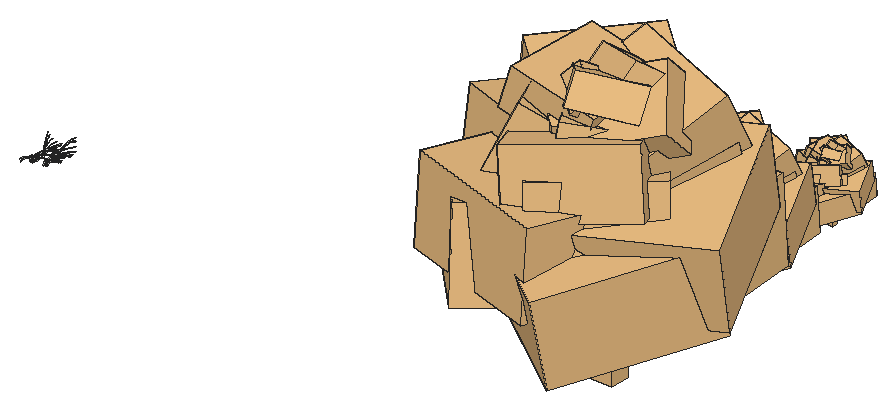
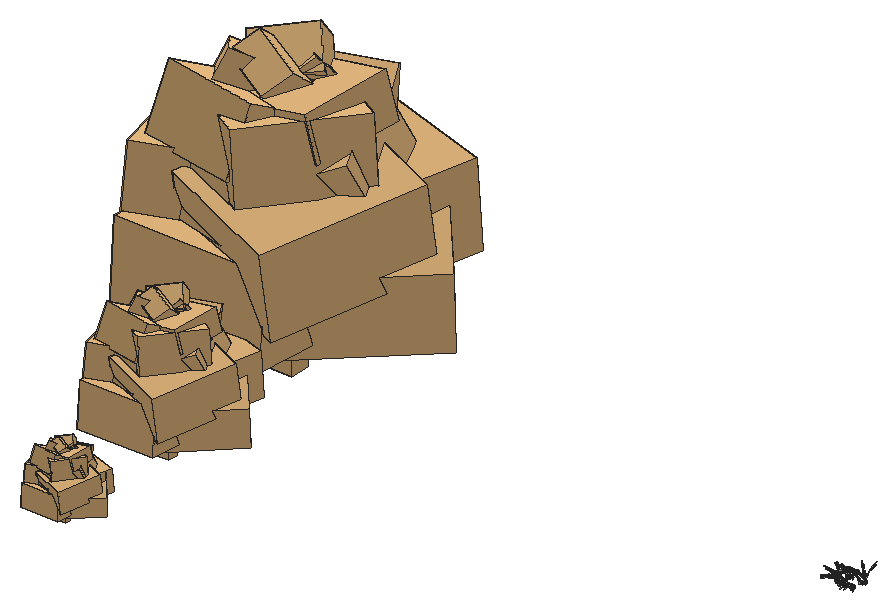
# SketchUp Ruby script. Lengths in inches.
U = 1.inch
M = Sketchup.active_model
def pt(a) = Geom::Point3d.new(a.map { |v| v * U })
def face(e, loops, mat)
  f = e.add_face(loops[0].map { |a| pt(a) })
  loops[1..].each { |l| e.add_face(l.map { |a| pt(a) }).erase! }
  f.material = f.back_material = mat if mat
  f
end
# faces: each face lists its corners as indices into pts; further lists are holes
def faces(e, pts, list, mat = nil) = list.each { |f| face(e, (f[0].is_a?(Array) ? f : [f]).map { |l| l.map { |i| pts[i] } }, mat) }
# xy, xz, yz: faces in a plane at the given z, y or x. An outline is a flat list of corners, or four numbers for a rectangle; further outlines are holes
def ring(l) = l.size == 4 ? [[l[0], l[1]], [l[2], l[1]], [l[2], l[3]], [l[0], l[3]]] : l.each_slice(2).to_a
def flat(e, list, mat, &to3) = list.each { |f| face(e, (f[0].is_a?(Array) ? f : [f]).map { |l| ring(l).map { |u, v| to3.(u, v) } }, mat) }
def xy(e, z, list, mat = nil) = flat(e, list, mat) { |x, y| [x, y, z] }
def xz(e, y, list, mat = nil) = flat(e, list, mat) { |x, z| [x, y, z] }
def yz(e, x, list, mat = nil) = flat(e, list, mat) { |y, z| [x, y, z] }
def lines(e, pts, list) = list.each { |a, b| e.add_line(pt(pts[a]), pt(pts[b])) }
# prism: a flat outline (further loops are holes) pulled along v
def prism(e, loops, v, mat = nil)
  f = face(e, loops, mat); d = Geom::Vector3d.new(v.map { |x| x * U })
  f.pushpull(f.normal.samedirection?(d) ? d.length : -d.length)
end
def box(e, o, s, mat = nil) = prism(e, [[o, [o[0] + s[0], o[1], o[2]], [o[0] + s[0], o[1] + s[1], o[2]], [o[0], o[1] + s[1], o[2]]]], [0, 0, s[2]], mat)
def at(x, y, z, deg = 0) = Geom::Transformation.translation(pt([x, y, z])) * Geom::Transformation.rotation(ORIGIN, Z_AXIS, deg.degrees)
def axes(o, x, y, z) = Geom::Transformation.new([*x, 0, *y, 0, *z, 0, *pt(o).to_a, 1])
def part(name) = M.definitions.add(name)
# library, detail: a bought-in or finely detailed component or shape, given as its bounding box
def library(name, o, s) = part(name).tap { |d| box(d.entities, o, s) }
def detail(e, o, s) = box(e.add_group.entities, o, s)
def put(e, d, t, mat = nil) = e.add_instance(d, t).tap { |i| i.material = mat if mat }
def group(e, t, mat = nil) = e.add_group.tap { |g| g.transformation = t; g.material = mat if mat }.entities
root = M.entities
c1 = library("Pine branch",[-164.19,86.97,62.64],[148.2,83.79,137.08])
c2 = part("Gruppe\#2")
detail(c2.entities,[0.71,-7.7,0],[22.57,19.31,263.85])
c3 = part("Kiefer Pine")
put(c3.entities,c1,axes([141.72,46.52,161.66],[-0.02916,-0.63772,0.00271],[0.15221,-0.00358,0.48358],[-0.6193,0.02915,0.11872]))
put(c3.entities,c1,axes([97.98,30.67,99.84],[-0.47537,-0.59297,0.00413],[0.14389,-0.11021,0.73807],[-0.57526,0.46243,0.1812]))
put(c3.entities,c1,axes([147.43,170.77,85.84],[0.66331,0.36209,0.08066],[-0.16152,0.13314,0.73061],[0.33395,-0.6548,0.19316]))
put(c3.entities,c1,axes([126.12,172.51,50.8],[0.58404,0.48629,0.00413],[-0.11903,0.13668,0.73807],[0.47151,-0.56784,0.1812]))
put(c3.entities,c1,axes([129.28,102.66,199.18],[0.3329,0.20176,-0.07756],[-0.04952,0.23763,0.27741],[0.2165,-0.24552,0.14305]))
put(c3.entities,c1,axes([28.39,91.46,58.6],[-0.71464,0.25212,0.05767],[-0.01186,-0.20123,0.73278],[0.25836,0.68814,0.19316]))
put(c3.entities,c1,axes([152.74,49.28,68.93],[0.33164,-0.67512,0.10878],[0.24998,0.23222,0.67911],[-0.63649,-0.26056,0.32339]))
put(c3.entities,c1,axes([-6.13,166.4,41.09],[-0.38774,0.8952,0.21972],[0.05521,-0.21538,0.97497],[0.92011,0.39016,0.03409]))
put(c3.entities,c1,axes([103.12,114.79,195.58],[-0.35402,0.16187,-0.07756],[-0.18541,-0.24864,0.1992],[0.04135,0.27092,0.22915]))
put(c3.entities,c1,axes([201.4375,150.2,7.87],[0.95266,-0.30403,0],[0.02078,0.06511,0.99766],[-0.30332,-0.95043,0.06835]))
put(c3.entities,c1,axes([149.14,-15.51,56.65],[-0.38076,-0.9108,0.15959],[0.00531,0.17044,0.98535],[-0.92466,0.37603,-0.06006]))
put(c3.entities,c1,axes([123.6,85.97,205.1],[0.23507,-0.19426,-0.06076],[0.16806,0.10538,0.1906],[-0.12474,-0.2241,0.1423]))
put(c3.entities,c1,axes([121.72,132.51,172.5],[0.36293,0.20783,-0.0399],[0.00027,0.10027,0.31921],[0.21403,-0.35254,0.06727]))
put(c3.entities,c1,axes([57.2,144.19,196.7],[-0.28797,0.37098,0.1914],[-0.03125,-0.30847,0.33516],[0.44369,0.21905,0.14782]))
put(c3.entities,c1,axes([93.55,232.34,18.61],[0.58552,0.78879,0.18704],[-0.06218,-0.18635,0.98051],[0.80827,-0.58574,-0.06006]))
put(c3.entities,c1,axes([33.34,105.32,91.71],[-0.72171,0.22385,0.08143],[-0.02606,-0.33247,0.68293],[0.23677,0.64572,0.32339]))
put(c3.entities,c1,axes([227.44,74.67,9.76],[0.6363,-0.72678,0.25867],[-0.14373,0.21775,0.96536],[-0.75793,-0.65144,0.03409]))
put(c3.entities,c1,axes([24.14,28.375,-27.51],[-1,0,0],[0,-0.06835,0.99766],[0,0.99766,0.06835]))
put(c3.entities,c2,at(97.66,98.27,0))
put(root,c3,axes([831.84,982.57,0],[0.375,0,0],[0,0.375,0],[0,0,0.375]))
put(root,c3,axes([795.14,752.84,0],[0.75,0,0],[0,0.75,0],[0,0,0.75]))
put(root,c3,axes([733.29,428.49,0],[1.5,0,0],[0,1.5,0],[0,0,1.5]))
g1 = group(root,at(81.27,576.14,0.02))
p = [[0.76,0.64,0],[0.34,0.29,0],[0,0,1.49],[0.14,0.12,2.99],[0.74,0.63,4.45],[1.8,1.53,5.86],
  [3.28,2.79,7.16],[5.16,4.39,8.33],[7.38,6.28,9.33],[9.89,8.41,10.15],[12.625,10.74,10.77],[15.52,13.2,11.16],
  [18.5,15.73,11.32],[21.5,18.28,11.24],[18.56,15.78,11.26],[15.65,13.31,11.05],[12.84,10.92,10.625],[10.19,8.66,9.99],
  [7.76,6.6,9.16],[5.61,4.77,8.16],[3.79,3.22,7.01],[2.33,1.98,5.73],[1.29,1.09,4.36],[0.67,0.57,2.93],
  [0.49,0.42,1.46]]
faces(g1,p,[[0,1,2,3,4,5,6,7,8,9,10,11,12,13,14,15,16,17,18,19,20,21,22,23,24]])
g2 = group(root,at(85.19,579.84,0.02))
p = [[20.78,-0.12,15.34],[23.91,-0.13,15.75],[20.875,-0.12,15.26],[17.94,-0.1,14.58],[15.15,-0.09,13.72],[12.52,-0.07,12.69],
  [10.09,-0.06,11.5],[7.88,-0.04,10.16],[5.93,-0.03,8.7],[4.24,-0.02,7.11],[2.85,-0.02,5.43],[1.76,-0.01,3.67],
  [0.99,-0.01,1.86],[0.54,0,0],[0,0,0],[0.37,0,1.9],[1.09,-0.01,3.76],[2.16,-0.01,5.57],
  [3.5625,-0.02,7.28],[5.28,-0.03,8.9],[7.3,-0.04,10.39],[9.58,-0.05,11.73],[12.11,-0.07,12.91],[14.84,-0.08,13.91],
  [17.74,-0.1,14.73]]
faces(g2,p,[[0,1,2,3,4,5,6,7,8,9,10,11,12,13,14,15,16,17,18,19,20,21,22,23,24]])
g3 = group(root,at(60.93,560.58,0.02))
p = [[0.99,-0.08,0],[0.44,-0.04,0],[0,0,1.49],[0.18,-0.01,2.99],[0.97,-0.08,4.45],[2.35,-0.19,5.86],
  [4.3,-0.35,7.16],[6.75,-0.55,8.33],[9.66,-0.78,9.33],[12.9375,-1.05,10.15],[16.52,-1.34,10.77],[20.31,-1.64,11.16],
  [24.21,-1.96,11.32],[28.13,-2.27,11.24],[24.28,-1.96,11.26],[20.48,-1.66,11.05],[16.8,-1.36,10.625],[13.33,-1.08,9.99],
  [10.15,-0.82,9.16],[7.34,-0.59,8.16],[4.95,-0.4,7.01],[3.05,-0.25,5.73],[1.68,-0.14,4.36],[0.87,-0.07,2.93],
  [0.64,-0.05,1.46]]
faces(g3,p,[[0,1,2,3,4,5,6,7,8,9,10,11,12,13,14,15,16,17,18,19,20,21,22,23,24]])
g4 = group(root,at(83.26,579.85,0.02))
p = [[20.78,-0.12,12.375],[23.91,-0.13,12.7],[20.875,-0.12,12.31],[17.94,-0.1,11.76],[15.15,-0.09,11.07],[12.52,-0.07,10.23],
  [10.09,-0.06,9.27],[7.88,-0.04,8.2],[5.93,-0.03,7.01],[4.24,-0.02,5.74],[2.85,-0.02,4.38],[1.76,-0.01,2.96],
  [0.99,-0.01,1.5],[0.54,0,0],[0,0,0],[0.37,0,1.53],[1.09,-0.01,3.03],[2.16,-0.01,4.49],
  [3.5625,-0.02,5.875],[5.28,-0.03,7.18],[7.3,-0.04,8.375],[9.58,-0.05,9.46],[12.11,-0.07,10.41],[14.84,-0.08,11.22],
  [17.74,-0.1,11.88]]
faces(g4,p,[[0,1,2,3,4,5,6,7,8,9,10,11,12,13,14,15,16,17,18,19,20,21,22,23,24]])
g5 = group(root,at(79.98,578.16,0.02))
p = [[0.92,-0.01,0],[0.41,0,0],[0,0,1.75],[0.17,0,3.51],[0.91,-0.01,5.24],[2.2,-0.01,6.89],
  [4.02,-0.02,8.42],[6.31,-0.04,9.8],[9.02,-0.05,10.98],[12.09,-0.07,11.95],[15.4375,-0.09,12.67],[18.98,-0.11,13.13],
  [22.625,-0.13,13.32],[26.29,-0.15,13.23],[22.69,-0.13,13.25],[19.14,-0.11,13],[15.7,-0.09,12.5],[12.45,-0.07,11.75],
  [9.49,-0.05,10.78],[6.86,-0.04,9.6],[4.63,-0.03,8.25],[2.85,-0.02,6.75],[1.57,-0.01,5.13],[0.8125,0,3.44],
  [0.6,0,1.72]]
faces(g5,p,[[0,1,2,3,4,5,6,7,8,9,10,11,12,13,14,15,16,17,18,19,20,21,22,23,24]])
g6 = group(root,at(66.33,560.42,0.02))
p = [[14.61,-14.77,15.34],[16.8125,-17,15.75],[14.68,-14.84,15.26],[12.62,-12.76,14.58],[10.65,-10.77,13.72],[8.8,-8.9,12.69],
  [7.09,-7.17,11.5],[5.54,-5.61,10.16],[4.17,-4.22,8.7],[2.98,-3.02,7.11],[2,-2.02,5.43],[1.24,-1.25,3.67],
  [0.69,-0.7,1.86],[0.38,-0.38,0],[0,0,0],[0.26,-0.26,1.9],[0.77,-0.77,3.76],[1.52,-1.54,5.57],
  [2.51,-2.53,7.28],[3.72,-3.76,8.9],[5.13,-5.19,10.39],[6.74,-6.8125,11.73],[8.51,-8.61,12.91],[10.43,-10.55,13.91],
  [12.47,-12.61,14.73]]
faces(g6,p,[[0,1,2,3,4,5,6,7,8,9,10,11,12,13,14,15,16,17,18,19,20,21,22,23,24]])
g7 = group(root,at(82.95,578.81,0.02))
p = [[0.52,0.77,0],[0.23,0.34,0],[0,0,1.75],[0.09,0.14,3.51],[0.51,0.75,5.24],[1.23,1.82,6.89],
  [2.25,3.33,8.42],[3.53,5.23,9.8],[5.05,7.48,10.98],[6.77,10.02,11.95],[8.64,12.8,12.67],[10.62,15.73,13.13],
  [12.66,18.75,13.32],[14.71,21.79,13.23],[12.7,18.81,13.25],[10.71,15.86,13],[8.78,13.01,12.5],[6.97,10.32,11.75],
  [5.31,7.86,10.78],[3.84,5.68,9.6],[2.59,3.84,8.25],[1.6,2.37,6.75],[0.88,1.3,5.13],[0.46,0.67,3.44],
  [0.33,0.49,1.72]]
faces(g7,p,[[0,1,2,3,4,5,6,7,8,9,10,11,12,13,14,15,16,17,18,19,20,21,22,23,24]])
g8 = group(root,at(64.97,561.8,0.02))
p = [[14.61,-14.77,12.375],[16.8125,-17,12.7],[14.68,-14.84,12.31],[12.62,-12.76,11.76],[10.65,-10.77,11.07],[8.8,-8.9,10.23],
  [7.09,-7.17,9.27],[5.54,-5.61,8.2],[4.17,-4.22,7.01],[2.98,-3.02,5.74],[2,-2.02,4.38],[1.24,-1.25,2.96],
  [0.69,-0.7,1.5],[0.38,-0.38,0],[0,0,0],[0.26,-0.26,1.53],[0.77,-0.77,3.03],[1.52,-1.54,4.49],
  [2.51,-2.53,5.875],[3.72,-3.76,7.18],[5.13,-5.19,8.375],[6.74,-6.8125,9.46],[8.51,-8.61,10.41],[10.43,-10.55,11.22],
  [12.47,-12.61,11.88]]
faces(g8,p,[[0,1,2,3,4,5,6,7,8,9,10,11,12,13,14,15,16,17,18,19,20,21,22,23,24]])
g9 = group(root,at(61.45,562.93,0.02))
p = [[0.65,-0.66,0],[0.29,-0.29,0],[0,0,1.75],[0.12,-0.12,3.51],[0.64,-0.64,5.24],[1.55,-1.5625,6.89],
  [2.82,-2.86,8.42],[4.4375,-4.49,9.8],[6.35,-6.42,10.98],[8.5,-8.6,11.95],[10.85,-10.98,12.67],[13.34,-13.49,13.13],
  [15.91,-16.09,13.32],[18.48,-18.69,13.23],[15.96,-16.14,13.25],[13.45,-13.61,13],[11.04,-11.16,12.5],[8.76,-8.86,11.75],
  [6.67,-6.74,10.78],[4.82,-4.875,9.6],[3.25,-3.29,8.25],[2.01,-2.03,6.75],[1.11,-1.12,5.13],[0.57,-0.58,3.44],
  [0.42,-0.42,1.72]]
faces(g9,p,[[0,1,2,3,4,5,6,7,8,9,10,11,12,13,14,15,16,17,18,19,20,21,22,23,24]])
g10 = group(root,at(84.27,579.48,0.02))
p = [[0.35,0.86,0],[0.16,0.38,0],[0,0,2.37],[0.0625,0.15,4.75],[0.35,0.84,7.08],[0.84,2.03,9.32],
  [1.53,3.71,11.39],[2.4,5.83,13.25],[3.4375,8.34,14.85],[4.61,11.18,16.15],[5.88,14.27,17.13],[7.23,17.55,17.75],
  [8.62,20.92,18.01],[10.02,24.3,17.89],[8.65,20.98,17.91],[7.29,17.69,17.58],[5.98,14.51,16.9],[4.75,11.52,15.89],
  [3.61,8.77,14.58],[2.61,6.34,12.99],[1.76,4.28,11.15],[1.09,2.64,9.125],[0.6,1.45,6.94],[0.31,0.75,4.66],
  [0.23,0.55,2.33]]
faces(g10,p,[[0,1,2,3,4,5,6,7,8,9,10,11,12,13,14,15,16,17,18,19,20,21,22,23,24]])
g11 = group(root,at(64.02,561.29,0.02))
p = [[0.91,0.18,0],[0.4,0.08,0],[0,0,1.75],[0.16,0.03,3.51],[0.89,0.17,5.24],[2.16,0.42,6.89],
  [3.94,0.76,8.42],[6.19,1.2,9.8],[8.86,1.72,10.98],[11.87,2.3,11.95],[15.16,2.94,12.67],[18.63,3.61,13.13],
  [22.21,4.31,13.32],[25.81,5.01,13.23],[22.28,4.32,13.25],[18.79,3.64,13],[15.41,2.99,12.5],[12.23,2.37,11.75],
  [9.3125,1.81,10.78],[6.73,1.31,9.6],[4.54,0.88,8.25],[2.8,0.54,6.75],[1.54,0.3,5.13],[0.8,0.16,3.44],
  [0.59,0.11,1.72]]
faces(g11,p,[[0,1,2,3,4,5,6,7,8,9,10,11,12,13,14,15,16,17,18,19,20,21,22,23,24]])
g12 = group(root,at(65.42,560.83,0.02))
p = [[0.85,0.36,0],[0.38,0.16,0],[0,0,2.37],[0.15,0.0625,4.75],[0.84,0.35,7.08],[2.03,0.85,9.32],
  [3.71,1.54,11.39],[5.83,2.42,13.25],[8.33,3.47,14.85],[11.16,4.65,16.15],[14.25,5.93,17.13],[17.52,7.29,17.75],
  [20.89,8.69,18.01],[24.27,10.1,17.89],[20.95,8.72,17.91],[17.67,7.35,17.58],[14.49,6.03,16.9],[11.5,4.79,15.89],
  [8.76,3.65,14.58],[6.33,2.63,12.99],[4.27,1.78,11.15],[2.63,1.1,9.125],[1.45,0.6,6.94],[0.75,0.3125,4.66],
  [0.55,0.23,2.33]]
faces(g12,p,[[0,1,2,3,4,5,6,7,8,9,10,11,12,13,14,15,16,17,18,19,20,21,22,23,24]])
g13 = group(root,at(83.21,584.52,0.02))
p = [[7.92,19.21,20.75],[9.11,22.11,21.3],[7.96,19.3,20.63],[6.84,16.59,19.72],[5.77,14.01,18.55],[4.77,11.58,17.16],
  [3.85,9.33,15.55],[3,7.29,13.74],[2.26,5.48,11.76],[1.62,3.92,9.62],[1.09,2.63,7.35],[0.67,1.625,4.97],
  [0.375,0.91,2.51],[0.21,0.5,0],[0,0,0],[0.14,0.34,2.57],[0.41,1.01,5.09],[0.82,2,7.53],
  [1.36,3.3,9.85],[2.01,4.89,12.03],[2.78,6.75,14.04],[3.65,8.86,15.86],[4.61,11.19,17.46],[5.65,13.72,18.82],
  [6.76,16.4,19.92]]
faces(g13,p,[[0,1,2,3,4,5,6,7,8,9,10,11,12,13,14,15,16,17,18,19,20,21,22,23,24]])
g14 = group(root,at(84.5625,577.8,0.02))
p = [[16.41,-12.74,15.34],[18.89,-14.66,15.75],[16.49,-12.8,15.26],[14.17,-11,14.58],[11.97,-9.29,13.72],[9.89,-7.68,12.69],
  [7.97,-6.1875,11.5],[6.23,-4.83,10.16],[4.68,-3.64,8.7],[3.35,-2.6,7.11],[2.25,-1.75,5.43],[1.39,-1.08,3.67],
  [0.78,-0.6,1.86],[0.43,-0.33,0],[0,0,0],[0.29,-0.22,1.9],[0.86,-0.67,3.76],[1.71,-1.32,5.57],
  [2.82,-2.1875,7.28],[4.17,-3.24,8.9],[5.77,-4.48,10.39],[7.57,-5.875,11.73],[9.5625,-7.42,12.91],[11.72,-9.1,13.91],
  [14.01,-10.88,14.73]]
faces(g14,p,[[0,1,2,3,4,5,6,7,8,9,10,11,12,13,14,15,16,17,18,19,20,21,22,23,24]])
g15 = group(root,at(78.09,577.63,0.02))
p = [[0.71,0.27,0],[0.31,0.12,0],[0,0,1.24],[0.13,0.05,2.49],[0.69,0.27,3.72],[1.68,0.65,4.89],
  [3.07,1.18,5.98],[4.83,1.85,6.95],[6.91,2.65,7.8],[9.26,3.55,8.48],[11.82,4.53,8.99],[14.53,5.57,9.32],
  [17.32,6.64,9.46],[20.125,7.72,9.39],[17.375,6.66,9.4],[14.65,5.62,9.23],[12.02,4.61,8.875],[9.54,3.66,8.35],
  [7.26,2.78,7.65],[5.25,2.01,6.82],[3.54,1.36,5.86],[2.18,0.84,4.79],[1.2,0.46,3.64],[0.625,0.24,2.45],
  [0.46,0.18,1.22]]
faces(g15,p,[[0,1,2,3,4,5,6,7,8,9,10,11,12,13,14,15,16,17,18,19,20,21,22,23,24]])
g16 = group(root,at(82.47,582.74,0.02))
p = [[7.92,19.21,16.73],[9.11,22.11,17.17],[7.96,19.3,16.64],[6.84,16.59,15.9],[5.77,14.01,14.96],[4.77,11.58,13.84],
  [3.85,9.33,12.54],[3,7.29,11.08],[2.26,5.48,9.48],[1.62,3.92,7.76],[1.09,2.63,5.92],[0.67,1.625,4.01],
  [0.375,0.91,2.02],[0.21,0.5,0],[0,0,0],[0.14,0.34,2.07],[0.41,1.01,4.1],[0.82,2,6.07],
  [1.36,3.3,7.94],[2.01,4.89,9.7],[2.78,6.75,11.33],[3.65,8.86,12.79],[4.61,11.19,14.08],[5.65,13.72,15.17],
  [6.76,16.4,16.0625]]
faces(g16,p,[[0,1,2,3,4,5,6,7,8,9,10,11,12,13,14,15,16,17,18,19,20,21,22,23,24]])
g17 = group(root,at(66.16,578.48,0.02))
p = [[0.07,0.81,0],[0.03,0.36,0],[0,0,1.23],[0.01,0.15,2.46],[0.0625,0.8,3.67],[0.16,1.9375,4.82],
  [0.29,3.54,5.89],[0.45,5.56,6.85],[0.64,7.95,7.68],[0.86,10.65,8.36],[1.1,13.6,8.86],[1.35,16.71,9.18],
  [1.61,19.92,9.32],[1.87,23.15,9.25],[1.62,19.98,9.27],[1.36,16.85,9.09],[1.12,13.82,8.74],[0.89,10.97,8.22],
  [0.68,8.35,7.54],[0.49,6.04,6.72],[0.33,4.08,5.77],[0.2,2.51,4.72],[0.11,1.38,3.59],[0.06,0.72,2.41],
  [0.04,0.53,1.2]]
faces(g17,p,[[0,1,2,3,4,5,6,7,8,9,10,11,12,13,14,15,16,17,18,19,20,21,22,23,24]])
g18 = group(root,at(68.24,565.14,0.02))
p = [[19.18,7.98,20.75],[22.08,9.1875,21.3],[19.27,8.02,20.63],[16.57,6.9,19.72],[13.98,5.82,18.55],[11.56,4.8125,17.16],
  [9.32,3.88,15.55],[7.28,3.03,13.74],[5.47,2.28,11.76],[3.92,1.63,9.62],[2.63,1.09,7.35],[1.625,0.68,4.97],
  [0.91,0.38,2.51],[0.5,0.21,0],[0,0,0],[0.34,0.14,2.57],[1.01,0.42,5.09],[1.99,0.83,7.53],
  [3.29,1.37,9.85],[4.88,2.03,12.03],[6.74,2.81,14.04],[8.85,3.68,15.86],[11.18,4.65,17.46],[13.7,5.7,18.82],
  [16.375,6.82,19.92]]
faces(g18,p,[[0,1,2,3,4,5,6,7,8,9,10,11,12,13,14,15,16,17,18,19,20,21,22,23,24]])
g19 = group(root,at(83.04,578.98,0.02))
p = [[16.41,-12.74,12.375],[18.89,-14.66,12.7],[16.49,-12.8,12.31],[14.17,-11,11.76],[11.97,-9.29,11.07],[9.89,-7.68,10.23],
  [7.97,-6.1875,9.27],[6.23,-4.83,8.2],[4.68,-3.64,7.01],[3.35,-2.6,5.74],[2.25,-1.75,4.38],[1.39,-1.08,2.96],
  [0.78,-0.6,1.5],[0.43,-0.33,0],[0,0,0],[0.29,-0.22,1.53],[0.86,-0.67,3.03],[1.71,-1.32,4.49],
  [2.82,-2.1875,5.875],[4.17,-3.24,7.18],[5.77,-4.48,8.375],[7.57,-5.875,9.46],[9.5625,-7.42,10.41],[11.72,-9.1,11.22],
  [14.01,-10.88,11.88]]
faces(g19,p,[[0,1,2,3,4,5,6,7,8,9,10,11,12,13,14,15,16,17,18,19,20,21,22,23,24]])
g20 = group(root,at(64.4375,559.43,0.02))
p = [[2.6,-20.61,15.34],[2.99,-23.72,15.75],[2.61,-20.71,15.26],[2.24,-17.8,14.58],[1.89,-15.03,13.72],[1.56,-12.42,12.69],
  [1.26,-10.01,11.5],[0.99,-7.82,10.16],[0.74,-5.88,8.7],[0.53,-4.21,7.11],[0.36,-2.83,5.43],[0.22,-1.74,3.67],
  [0.125,-0.98,1.86],[0.07,-0.54,0],[0,0,0],[0.05,-0.36,1.9],[0.14,-1.08,3.76],[0.27,-2.14,5.57],
  [0.45,-3.54,7.28],[0.66,-5.24,8.9],[0.91,-7.24,10.39],[1.2,-9.51,11.73],[1.51,-12.01,12.91],[1.85,-14.72,13.91],
  [2.22,-17.6,14.73]]
faces(g20,p,[[0,1,2,3,4,5,6,7,8,9,10,11,12,13,14,15,16,17,18,19,20,21,22,23,24]])
g21 = group(root,at(79.64,581.62,0.02))
p = [[0.78,-0.61,0],[0.35,-0.27,0],[0,0,1.49],[0.14,-0.11,2.99],[0.77,-0.6,4.45],[1.87,-1.45,5.86],
  [3.41,-2.64,7.16],[5.35,-4.15,8.33],[7.65,-5.94,9.33],[10.25,-7.96,10.15],[13.09,-10.16,10.77],[16.09,-12.49,11.16],
  [19.18,-14.89,11.32],[22.29,-17.3,11.24],[19.24,-14.9375,11.26],[16.23,-12.6,11.05],[13.3125,-10.33,10.625],[10.5625,-8.2,9.99],
  [8.04,-6.24,9.16],[5.8125,-4.51,8.16],[3.93,-3.05,7.01],[2.42,-1.88,5.73],[1.33,-1.04,4.36],[0.69,-0.54,2.93],
  [0.51,-0.39,1.46]]
faces(g21,p,[[0,1,2,3,4,5,6,7,8,9,10,11,12,13,14,15,16,17,18,19,20,21,22,23,24]])
g22 = group(root,at(66.3,582.92,0.02))
p = [[12.16,12.02,12.63],[13.99,13.84,12.96],[12.22,12.08,12.56],[10.5,10.38,12],[8.86,8.77,11.29],[7.33,7.25,10.44],
  [5.9,5.84,9.46],[4.61,4.5625,8.36],[3.47,3.43,7.16],[2.48,2.46,5.85],[1.67,1.65,4.47],[1.03,1.02,3.02],
  [0.58,0.57,1.53],[0.32,0.3125,0],[0,0,0],[0.21,0.21,1.5625],[0.64,0.63,3.1],[1.26,1.25,4.58],
  [2.09,2.0625,6],[3.09,3.06,7.32],[4.27,4.22,8.55],[5.61,5.55,9.65],[7.08,7.01,10.625],[8.68,8.59,11.45],
  [10.38,10.27,12.12]]
faces(g22,p,[[0,1,2,3,4,5,6,7,8,9,10,11,12,13,14,15,16,17,18,19,20,21,22,23,24]])
g23 = group(root,at(81.09,560.69,0.02))
p = [[0.67,0.57,0],[0.3,0.25,0],[0,0,1.32],[0.12,0.1,2.64],[0.66,0.56,3.94],[1.59,1.35,5.18],
  [2.91,2.47,6.33],[4.57,3.88,7.37],[6.53,5.55,8.26],[8.75,7.44,8.99],[11.17,9.5,9.53],[13.73,11.68,9.875],
  [16.37,13.92,10.02],[19.02,16.18,9.95],[16.42,13.97,9.96],[13.85,11.78,9.78],[11.36,9.66,9.4],[9.01,7.67,8.84],
  [6.86,5.84,8.11],[4.96,4.22,7.22],[3.35,2.85,6.2],[2.07,1.76,5.07],[1.14,0.97,3.86],[0.59,0.5,2.59],
  [0.43,0.37,1.29]]
faces(g23,p,[[0,1,2,3,4,5,6,7,8,9,10,11,12,13,14,15,16,17,18,19,20,21,22,23,24]])
g24 = group(root,at(59.74,563.88,0.02))
p = [[0.69,-0.31,0],[0.31,-0.14,0],[0,0,1.24],[0.125,-0.06,2.49],[0.68,-0.3,3.72],[1.65,-0.73,4.89],
  [3.01,-1.34,5.98],[4.73,-2.11,6.95],[6.76,-3.01,7.8],[9.06,-4.04,8.48],[11.5625,-5.15,8.99],[14.21,-6.33,9.32],
  [16.94,-7.55,9.46],[19.6875,-8.77,9.39],[17,-7.58,9.4],[14.33,-6.39,9.23],[11.76,-5.24,8.875],[9.33,-4.16,8.35],
  [7.1,-3.17,7.65],[5.14,-2.29,6.82],[3.47,-1.55,5.86],[2.14,-0.95,4.79],[1.18,-0.52,3.64],[0.61,-0.27,2.45],
  [0.45,-0.2,1.22]]
faces(g24,p,[[0,1,2,3,4,5,6,7,8,9,10,11,12,13,14,15,16,17,18,19,20,21,22,23,24]])
g25 = group(root,at(66.45,564.4,0.02))
p = [[19.18,7.98,16.73],[22.08,9.1875,17.17],[19.27,8.02,16.64],[16.57,6.9,15.9],[13.98,5.82,14.96],[11.56,4.8125,13.84],
  [9.32,3.88,12.54],[7.28,3.03,11.08],[5.47,2.28,9.48],[3.92,1.63,7.76],[2.63,1.09,5.92],[1.625,0.68,4.01],
  [0.91,0.38,2.02],[0.5,0.21,0],[0,0,0],[0.34,0.14,2.07],[1.01,0.42,4.1],[1.99,0.83,6.07],
  [3.29,1.37,7.94],[4.88,2.03,9.7],[6.74,2.81,11.33],[8.85,3.68,12.79],[11.18,4.65,14.08],[13.7,5.7,15.17],
  [16.375,6.82,16.0625]]
faces(g25,p,[[0,1,2,3,4,5,6,7,8,9,10,11,12,13,14,15,16,17,18,19,20,21,22,23,24]])
g26 = group(root,at(84.5625,563.97,0.02))
p = [[18.39,-0.1,13.58],[21.16,-0.12,13.9375],[18.47,-0.1,13.5],[15.88,-0.09,12.9],[13.41,-0.08,12.14],[11.08,-0.0625,11.23],
  [8.93,-0.05,10.18],[6.98,-0.04,8.99],[5.25,-0.03,7.7],[3.75,-0.02,6.29],[2.52,-0.01,4.81],[1.56,-0.01,3.25],
  [0.87,0,1.64],[0.48,0,0],[0,0,0],[0.32,0,1.68],[0.96,-0.01,3.33],[1.91,-0.01,4.92],
  [3.15,-0.02,6.45],[4.68,-0.03,7.875],[6.46,-0.04,9.19],[8.48,-0.05,10.38],[10.71,-0.06,11.43],[13.13,-0.07,12.3125],
  [15.7,-0.09,13.03]]
faces(g26,p,[[0,1,2,3,4,5,6,7,8,9,10,11,12,13,14,15,16,17,18,19,20,21,22,23,24]])
g27 = group(root,at(65.17,581.8,0.02))
p = [[12.16,12.02,10.18],[13.99,13.84,10.45],[12.22,12.08,10.13],[10.5,10.38,9.68],[8.86,8.77,9.11],[7.33,7.25,8.42],
  [5.9,5.84,7.63],[4.61,4.5625,6.75],[3.47,3.43,5.77],[2.48,2.46,4.72],[1.67,1.65,3.61],[1.03,1.02,2.4375],
  [0.58,0.57,1.23],[0.32,0.3125,0],[0,0,0],[0.21,0.21,1.26],[0.64,0.63,2.5],[1.26,1.25,3.69],
  [2.09,2.0625,4.83],[3.09,3.06,5.91],[4.27,4.22,6.89],[5.61,5.55,7.78],[7.08,7.01,8.57],[8.68,8.59,9.24],
  [10.38,10.27,9.78]]
faces(g27,p,[[0,1,2,3,4,5,6,7,8,9,10,11,12,13,14,15,16,17,18,19,20,21,22,23,24]])
g28 = group(root,at(64.2,561.34,0.02))
p = [[2.6,-20.61,12.375],[2.99,-23.72,12.7],[2.61,-20.71,12.31],[2.24,-17.8,11.76],[1.89,-15.03,11.07],[1.56,-12.42,10.23],
  [1.26,-10.01,9.27],[0.99,-7.82,8.2],[0.74,-5.88,7.01],[0.53,-4.21,5.74],[0.36,-2.83,4.38],[0.22,-1.74,2.96],
  [0.125,-0.98,1.5],[0.07,-0.54,0],[0,0,0],[0.05,-0.36,1.53],[0.14,-1.08,3.03],[0.27,-2.14,4.49],
  [0.45,-3.54,5.875],[0.66,-5.24,7.18],[0.91,-7.24,8.375],[1.2,-9.51,9.46],[1.51,-12.01,10.41],[1.85,-14.72,11.22],
  [2.22,-17.6,11.88]]
faces(g28,p,[[0,1,2,3,4,5,6,7,8,9,10,11,12,13,14,15,16,17,18,19,20,21,22,23,24]])
g29 = group(root,at(64.24,578.9,0.02))
p = [[0.54,0.54,0],[0.24,0.24,0],[0,0,1.44],[0.1,0.1,2.89],[0.53,0.52,4.3125],[1.29,1.27,5.67],
  [2.35,2.32,6.93],[3.69,3.65,8.0625],[5.28,5.22,9.04],[7.08,7,9.83],[9.03,8.93,10.43],[11.11,10.98,10.81],
  [13.24,13.09,10.96],[15.38,15.21,10.89],[13.28,13.13,10.9],[11.2,11.07,10.7],[9.1875,9.08,10.29],[7.29,7.21,9.67],
  [5.55,5.49,8.875],[4.01,3.97,7.9],[2.71,2.68,6.79],[1.67,1.65,5.55],[0.92,0.91,4.22],[0.48,0.47,2.83],
  [0.35,0.35,1.42]]
faces(g29,p,[[0,1,2,3,4,5,6,7,8,9,10,11,12,13,14,15,16,17,18,19,20,21,22,23,24]])
g30 = group(root,at(63.66,565.62,0.02))
p = [[0.125,-0.99,0],[0.06,-0.4375,0],[0,0,1.49],[0.02,-0.18,2.99],[0.12,-0.96,4.45],[0.3,-2.34,5.86],
  [0.54,-4.28,7.16],[0.85,-6.72,8.33],[1.21,-9.61,9.33],[1.62,-12.88,10.15],[2.07,-16.44,10.77],[2.55,-20.21,11.16],
  [3.03,-24.1,11.32],[3.53,-28,11.24],[3.04,-24.17,11.26],[2.57,-20.38,11.05],[2.11,-16.72,10.625],[1.67,-13.27,9.99],
  [1.27,-10.1,9.16],[0.92,-7.3,8.16],[0.62,-4.93,7.01],[0.38,-3.04,5.73],[0.21,-1.67,4.36],[0.11,-0.87,2.93],
  [0.08,-0.64,1.46]]
faces(g30,p,[[0,1,2,3,4,5,6,7,8,9,10,11,12,13,14,15,16,17,18,19,20,21,22,23,24]])
g31 = group(root,at(82.85,563.98,0.02))
p = [[18.39,-0.1,10.95],[21.16,-0.12,11.24],[18.47,-0.1,10.89],[15.88,-0.09,10.41],[13.41,-0.08,9.79],[11.08,-0.0625,9.06],
  [8.93,-0.05,8.21],[6.98,-0.04,7.25],[5.25,-0.03,6.21],[3.75,-0.02,5.08],[2.52,-0.01,3.875],[1.56,-0.01,2.62],
  [0.87,0,1.32],[0.48,0,0],[0,0,0],[0.32,0,1.36],[0.96,-0.01,2.69],[1.91,-0.01,3.97],
  [3.15,-0.02,5.2],[4.68,-0.03,6.35],[6.46,-0.04,7.41],[8.48,-0.05,8.37],[10.71,-0.06,9.21],[13.13,-0.07,9.93],
  [15.7,-0.09,10.51]]
faces(g31,p,[[0,1,2,3,4,5,6,7,8,9,10,11,12,13,14,15,16,17,18,19,20,21,22,23,24]])
g32 = group(root,at(65.59,581.02,0.02))
p = [[-0.14,0.75,0],[-0.0625,0.33,0],[0,0,1.44],[-0.03,0.13,2.89],[-0.14,0.73,4.3125],[-0.34,1.78,5.67],
  [-0.63,3.24,6.93],[-0.99,5.1,8.0625],[-1.41,7.29,9.04],[-1.9,9.77,9.83],[-2.42,12.47,10.43],[-2.97,15.33,10.81],
  [-3.55,18.28,10.96],[-4.12,21.24,10.89],[-3.56,18.33,10.9],[-3,15.46,10.7],[-2.46,12.68,10.29],[-1.95,10.0625,9.67],
  [-1.49,7.66,8.875],[-1.07,5.54,7.9],[-0.73,3.74,6.79],[-0.45,2.31,5.55],[-0.25,1.27,4.22],[-0.13,0.66,2.83],
  [-0.09,0.48,1.42]]
faces(g32,p,[[0,1,2,3,4,5,6,7,8,9,10,11,12,13,14,15,16,17,18,19,20,21,22,23,24]])
g33 = group(root,at(79.94,562.48,0.02))
p = [[0.82,0,0],[0.36,0,0],[0,0,1.55],[0.15,0,3.11],[0.8,0,4.64],[1.95,-0.01,6.1],
  [3.55,-0.02,7.45],[5.58,-0.03,8.67],[7.99,-0.04,9.72],[10.7,-0.06,10.57],[13.66,-0.08,11.21],[16.79,-0.09,11.62],
  [20.02,-0.11,11.79],[23.26,-0.13,11.71],[20.08,-0.11,11.72],[16.93,-0.1,11.5],[13.89,-0.08,11.0625],[11.02,-0.0625,10.4],
  [8.39,-0.05,9.54],[6.07,-0.03,8.5],[4.1,-0.02,7.3],[2.53,-0.01,5.97],[1.39,-0.01,4.54],[0.72,0,3.05],
  [0.53,0,1.52]]
faces(g33,p,[[0,1,2,3,4,5,6,7,8,9,10,11,12,13,14,15,16,17,18,19,20,21,22,23,24]])
g34 = group(root,at(65.96,582.17,0.02))
p = [[-0.29,0.7,0],[-0.13,0.3125,0],[0,0,1.95],[-0.05,0.125,3.91],[-0.29,0.6875,5.83],[-0.7,1.67,7.67],
  [-1.27,3.05,9.37],[-2,4.79,10.9],[-2.85,6.86,12.22],[-3.82,9.1875,13.3],[-4.88,11.73,14.1],[-6,14.42,14.61],
  [-7.16,17.19,14.82],[-8.3125,19.97,14.72],[-7.18,17.24,14.74],[-6.05,14.54,14.47],[-4.96,11.93,13.91],[-3.9375,9.46,13.08],
  [-3,7.21,12],[-2.17,5.21,10.6875],[-1.46,3.52,9.18],[-0.9,2.17,7.51],[-0.5,1.19,5.71],[-0.26,0.62,3.83],
  [-0.1875,0.45,1.91]]
faces(g34,p,[[0,1,2,3,4,5,6,7,8,9,10,11,12,13,14,15,16,17,18,19,20,21,22,23,24]])
g35 = group(root,at(82.57,563.0625,0.02))
p = [[0.46,0.68,0],[0.2,0.3,0],[0,0,1.55],[0.08,0.12,3.11],[0.45,0.66,4.64],[1.09,1.61,6.1],
  [1.99,2.95,7.45],[3.125,4.63,8.67],[4.47,6.62,9.72],[5.99,8.87,10.57],[7.64,11.32,11.21],[9.4,13.92,11.62],
  [11.2,16.59,11.79],[13.02,19.28,11.71],[11.24,16.64,11.72],[9.47,14.04,11.5],[7.77,11.51,11.0625],[6.17,9.14,10.4],
  [4.7,6.96,9.54],[3.39,5.03,8.5],[2.29,3.4,7.3],[1.41,2.09,5.97],[0.78,1.15,4.54],[0.4,0.6,3.05],
  [0.3,0.4375,1.52]]
faces(g35,p,[[0,1,2,3,4,5,6,7,8,9,10,11,12,13,14,15,16,17,18,19,20,21,22,23,24]])
g36 = group(root,at(83.74,563.65,0.02))
p = [[0.3125,0.76,0],[0.14,0.34,0],[0,0,2.1],[0.06,0.14,4.2],[0.31,0.74,6.27],[0.74,1.8,8.24],
  [1.35,3.29,10.08],[2.13,5.16,11.72],[3.04,7.38,13.14],[4.08,9.89,14.3],[5.21,12.63,15.16],[6.4,15.53,15.71],
  [7.63,18.51,15.9375],[8.86,21.51,15.83],[7.65,18.57,15.85],[6.45,15.66,15.56],[5.29,12.84,14.96],[4.2,10.19,14.07],
  [3.2,7.76,12.9],[2.3125,5.61,11.49],[1.5625,3.79,9.87],[0.96,2.33,8.07],[0.53,1.29,6.14],[0.27,0.67,4.12],
  [0.2,0.49,2.06]]
faces(g36,p,[[0,1,2,3,4,5,6,7,8,9,10,11,12,13,14,15,16,17,18,19,20,21,22,23,24]])
g37 = group(root,at(78.07,576.12,0.02))
p = [[0.73,-0.57,0],[0.32,-0.25,0],[0,0,1.75],[0.13,-0.1,3.51],[0.72,-0.56,5.24],[1.74,-1.35,6.89],
  [3.17,-2.46,8.42],[4.98,-3.87,9.8],[7.13,-5.53,10.98],[9.55,-7.42,11.95],[12.19,-9.47,12.67],[14.99,-11.64,13.13],
  [17.87,-13.875,13.32],[20.76,-16.12,13.23],[17.93,-13.92,13.25],[15.12,-11.73,13],[12.4,-9.625,12.5],[9.84,-7.64,11.75],
  [7.49,-5.82,10.78],[5.42,-4.2,9.6],[3.66,-2.84,8.25],[2.25,-1.75,6.75],[1.24,-0.96,5.13],[0.64,-0.5,3.44],
  [0.47,-0.37,1.72]]
faces(g37,p,[[0,1,2,3,4,5,6,7,8,9,10,11,12,13,14,15,16,17,18,19,20,21,22,23,24]])
g38 = group(root,at(74.27,585.01,0.02))
p = [[18.35,-9.75,14.56],[21.11,-11.23,14.94],[18.43,-9.8,14.48],[15.84,-8.42,13.83],[13.375,-7.11,13.02],[11.05,-5.88,12.04],
  [8.91,-4.74,10.91],[6.96,-3.7,9.64],[5.23,-2.78,8.25],[3.75,-1.99,6.75],[2.51,-1.34,5.15],[1.55,-0.83,3.49],
  [0.87,-0.46,1.76],[0.48,-0.25,0],[0,0,0],[0.32,-0.17,1.8],[0.96,-0.51,3.57],[1.91,-1.01,5.28],
  [3.15,-1.67,6.91],[4.67,-2.48,8.44],[6.45,-3.43,9.85],[8.46,-4.5,11.13],[10.6875,-5.68,12.25],[13.1,-6.97,13.2],
  [15.66,-8.33,13.97]]
faces(g38,p,[[0,1,2,3,4,5,6,7,8,9,10,11,12,13,14,15,16,17,18,19,20,21,22,23,24]])
g39 = group(root,at(62.41,584.49,0.02))
p = [[-6.57,15.79,17.08],[-7.5625,18.17,17.53],[-6.6,15.86,16.98],[-5.68,13.63,16.23],[-4.79,11.51,15.27],[-3.96,9.51,14.125],
  [-3.19,7.67,12.8],[-2.49,5.99,11.3125],[-1.875,4.5,9.68],[-1.34,3.22,7.92],[-0.9,2.16,6.05],[-0.56,1.34,4.09],
  [-0.3125,0.75,2.07],[-0.17,0.41,0],[0,0,0],[-0.12,0.28,2.11],[-0.34,0.83,4.1875],[-0.68,1.64,6.19],
  [-1.13,2.71,8.11],[-1.67,4.02,9.9],[-2.31,5.55,11.56],[-3.03,7.28,13.05],[-3.83,9.2,14.37],[-4.69,11.27,15.49],
  [-5.61,13.48,16.39]]
faces(g39,p,[[0,1,2,3,4,5,6,7,8,9,10,11,12,13,14,15,16,17,18,19,20,21,22,23,24]])
g40 = group(root,at(67.12,581.36,0.02))
p = [[16.97,2.14,12.63],[19.53,2.46,12.96],[17.05,2.15,12.56],[14.65,1.85,12],[12.37,1.56,11.29],[10.22,1.29,10.44],
  [8.24,1.04,9.46],[6.4375,0.8125,8.36],[4.84,0.61,7.16],[3.46,0.4375,5.85],[2.33,0.29,4.47],[1.4375,0.18,3.02],
  [0.81,0.1,1.53],[0.44,0.06,0],[0,0,0],[0.3,0.04,1.5625],[0.89,0.11,3.1],[1.76,0.22,4.58],
  [2.91,0.37,6],[4.32,0.54,7.32],[5.96,0.75,8.55],[7.83,0.99,9.65],[9.89,1.25,10.625],[12.11,1.53,11.45],
  [14.48,1.82,12.12]]
faces(g40,p,[[0,1,2,3,4,5,6,7,8,9,10,11,12,13,14,15,16,17,18,19,20,21,22,23,24]])
